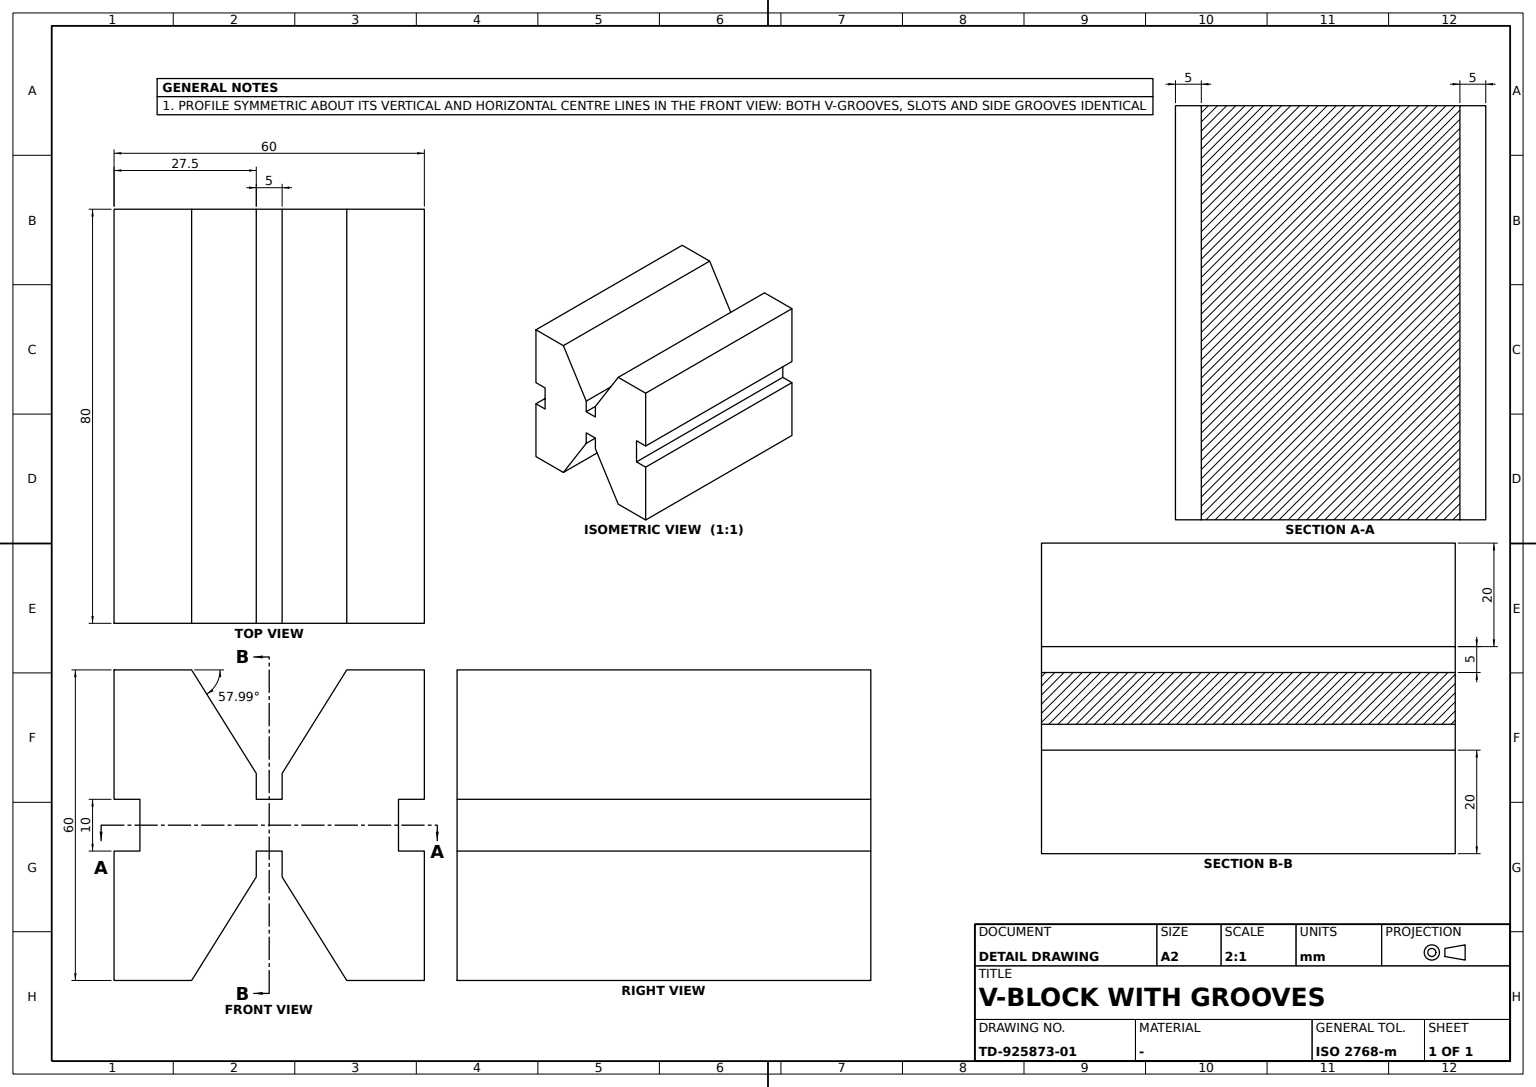
ISO-10303-21;
HEADER;
FILE_DESCRIPTION((''),'2;1');
FILE_NAME('','',(''),(''),'','','');
FILE_SCHEMA(('AUTOMOTIVE_DESIGN'));
ENDSEC;
DATA;
#1=APPLICATION_CONTEXT('');
#2=PRODUCT_CONTEXT('',#1,'mechanical');
#3=PRODUCT('','','',(#2));
#4=PRODUCT_DEFINITION_FORMATION('','',#3);
#5=PRODUCT_DEFINITION_CONTEXT('',#1,'design');
#6=PRODUCT_DEFINITION('','',#4,#5);
#7=PRODUCT_DEFINITION_SHAPE('','',#6);
#8=(LENGTH_UNIT()NAMED_UNIT(*)SI_UNIT(.MILLI.,.METRE.));
#9=(NAMED_UNIT(*)PLANE_ANGLE_UNIT()SI_UNIT($,.RADIAN.));
#10=(NAMED_UNIT(*)SI_UNIT($,.STERADIAN.)SOLID_ANGLE_UNIT());
#11=UNCERTAINTY_MEASURE_WITH_UNIT(LENGTH_MEASURE(1.E-05),#8,'distance_accuracy_value','');
#12=(GEOMETRIC_REPRESENTATION_CONTEXT(3)GLOBAL_UNCERTAINTY_ASSIGNED_CONTEXT((#11))GLOBAL_UNIT_ASSIGNED_CONTEXT((#8,#9,#10))REPRESENTATION_CONTEXT('',''));
#13=CARTESIAN_POINT('',(-40.,-2.5,10.));
#14=VERTEX_POINT('',#13);
#15=CARTESIAN_POINT('',(40.,-2.5,10.));
#16=VERTEX_POINT('',#15);
#17=CARTESIAN_POINT('',(0.,-2.5,10.));
#18=DIRECTION('',(1.,0.,0.));
#19=VECTOR('',#18,1000.);
#20=LINE('',#17,#19);
#21=EDGE_CURVE('',#14,#16,#20,.T.);
#22=ORIENTED_EDGE('',*,*,#21,.F.);
#23=CARTESIAN_POINT('',(-40.,-15.,30.));
#24=VERTEX_POINT('',#23);
#25=CARTESIAN_POINT('',(-40.,-8.75,20.));
#26=DIRECTION('',(0.,0.52999894,-0.847998304));
#27=VECTOR('',#26,1000.);
#28=LINE('',#25,#27);
#29=EDGE_CURVE('',#24,#14,#28,.T.);
#30=ORIENTED_EDGE('',*,*,#29,.F.);
#31=CARTESIAN_POINT('',(40.,-15.,30.));
#32=VERTEX_POINT('',#31);
#33=CARTESIAN_POINT('',(0.,-15.,30.));
#34=LINE('',#33,#19);
#35=EDGE_CURVE('',#24,#32,#34,.T.);
#36=ORIENTED_EDGE('',*,*,#35,.T.);
#37=CARTESIAN_POINT('',(40.,-8.75,20.));
#38=LINE('',#37,#27);
#39=EDGE_CURVE('',#32,#16,#38,.T.);
#40=ORIENTED_EDGE('',*,*,#39,.T.);
#41=EDGE_LOOP('',(#22,#30,#36,#40));
#42=FACE_OUTER_BOUND('',#41,.T.);
#43=DIRECTION('',(0.,0.847998304,0.52999894));
#44=DIRECTION('',(0.,-0.52999894,0.847998304));
#45=AXIS2_PLACEMENT_3D('',#17,#43,#44);
#46=PLANE('',#45);
#47=ADVANCED_FACE('',(#42),#46,.T.);
#48=CARTESIAN_POINT('',(-40.,-15.,-30.));
#49=VERTEX_POINT('',#48);
#50=CARTESIAN_POINT('',(40.,-15.,-30.));
#51=VERTEX_POINT('',#50);
#52=CARTESIAN_POINT('',(0.,-15.,-30.));
#53=LINE('',#52,#19);
#54=EDGE_CURVE('',#49,#51,#53,.T.);
#55=ORIENTED_EDGE('',*,*,#54,.T.);
#56=CARTESIAN_POINT('',(40.,-30.,-30.));
#57=VERTEX_POINT('',#56);
#58=CARTESIAN_POINT('',(40.,-22.5,-30.));
#59=DIRECTION('',(0.,-1.,0.));
#60=VECTOR('',#59,1000.);
#61=LINE('',#58,#60);
#62=EDGE_CURVE('',#51,#57,#61,.T.);
#63=ORIENTED_EDGE('',*,*,#62,.T.);
#64=CARTESIAN_POINT('',(-40.,-30.,-30.));
#65=VERTEX_POINT('',#64);
#66=CARTESIAN_POINT('',(0.,-30.,-30.));
#67=LINE('',#66,#19);
#68=EDGE_CURVE('',#65,#57,#67,.T.);
#69=ORIENTED_EDGE('',*,*,#68,.F.);
#70=CARTESIAN_POINT('',(-40.,-22.5,-30.));
#71=LINE('',#70,#60);
#72=EDGE_CURVE('',#49,#65,#71,.T.);
#73=ORIENTED_EDGE('',*,*,#72,.F.);
#74=EDGE_LOOP('',(#55,#63,#69,#73));
#75=FACE_OUTER_BOUND('',#74,.T.);
#76=CARTESIAN_POINT('',(0.,30.,-30.));
#77=DIRECTION('',(0.,0.,1.));
#78=AXIS2_PLACEMENT_3D('',#76,#77,#59);
#79=PLANE('',#78);
#80=ADVANCED_FACE('',(#75),#79,.F.);
#81=CARTESIAN_POINT('',(-40.,2.5,10.));
#82=VERTEX_POINT('',#81);
#83=CARTESIAN_POINT('',(-40.,2.5,5.));
#84=VERTEX_POINT('',#83);
#85=CARTESIAN_POINT('',(-40.,2.5,7.5));
#86=DIRECTION('',(0.,0.,-1.));
#87=VECTOR('',#86,1000.);
#88=LINE('',#85,#87);
#89=EDGE_CURVE('',#82,#84,#88,.T.);
#90=ORIENTED_EDGE('',*,*,#89,.T.);
#91=CARTESIAN_POINT('',(40.,2.5,5.));
#92=VERTEX_POINT('',#91);
#93=CARTESIAN_POINT('',(0.,2.5,5.));
#94=LINE('',#93,#19);
#95=EDGE_CURVE('',#84,#92,#94,.T.);
#96=ORIENTED_EDGE('',*,*,#95,.T.);
#97=CARTESIAN_POINT('',(40.,2.5,10.));
#98=VERTEX_POINT('',#97);
#99=CARTESIAN_POINT('',(40.,2.5,7.5));
#100=LINE('',#99,#87);
#101=EDGE_CURVE('',#98,#92,#100,.T.);
#102=ORIENTED_EDGE('',*,*,#101,.F.);
#103=CARTESIAN_POINT('',(0.,2.5,10.));
#104=LINE('',#103,#19);
#105=EDGE_CURVE('',#82,#98,#104,.T.);
#106=ORIENTED_EDGE('',*,*,#105,.F.);
#107=EDGE_LOOP('',(#90,#96,#102,#106));
#108=FACE_OUTER_BOUND('',#107,.T.);
#109=DIRECTION('',(0.,1.,0.));
#110=AXIS2_PLACEMENT_3D('',#93,#109,#77);
#111=PLANE('',#110);
#112=ADVANCED_FACE('',(#108),#111,.F.);
#113=CARTESIAN_POINT('',(-40.,-2.5,5.));
#114=VERTEX_POINT('',#113);
#115=CARTESIAN_POINT('',(-40.,0.,5.));
#116=VECTOR('',#109,1000.);
#117=LINE('',#115,#116);
#118=EDGE_CURVE('',#114,#84,#117,.T.);
#119=ORIENTED_EDGE('',*,*,#118,.F.);
#120=CARTESIAN_POINT('',(40.,-2.5,5.));
#121=VERTEX_POINT('',#120);
#122=CARTESIAN_POINT('',(0.,-2.5,5.));
#123=LINE('',#122,#19);
#124=EDGE_CURVE('',#114,#121,#123,.T.);
#125=ORIENTED_EDGE('',*,*,#124,.T.);
#126=CARTESIAN_POINT('',(40.,0.,5.));
#127=LINE('',#126,#116);
#128=EDGE_CURVE('',#121,#92,#127,.T.);
#129=ORIENTED_EDGE('',*,*,#128,.T.);
#130=ORIENTED_EDGE('',*,*,#95,.F.);
#131=EDGE_LOOP('',(#119,#125,#129,#130));
#132=FACE_OUTER_BOUND('',#131,.T.);
#133=CARTESIAN_POINT('',(0.,0.,5.));
#134=AXIS2_PLACEMENT_3D('',#133,#86,#109);
#135=PLANE('',#134);
#136=ADVANCED_FACE('',(#132),#135,.F.);
#137=CARTESIAN_POINT('',(-40.,-30.,-5.));
#138=VERTEX_POINT('',#137);
#139=CARTESIAN_POINT('',(-40.,-25.,-5.));
#140=VERTEX_POINT('',#139);
#141=CARTESIAN_POINT('',(-40.,-27.5,-5.));
#142=LINE('',#141,#116);
#143=EDGE_CURVE('',#138,#140,#142,.T.);
#144=ORIENTED_EDGE('',*,*,#143,.F.);
#145=CARTESIAN_POINT('',(40.,-30.,-5.));
#146=VERTEX_POINT('',#145);
#147=CARTESIAN_POINT('',(0.,-30.,-5.));
#148=LINE('',#147,#19);
#149=EDGE_CURVE('',#138,#146,#148,.T.);
#150=ORIENTED_EDGE('',*,*,#149,.T.);
#151=CARTESIAN_POINT('',(40.,-25.,-5.));
#152=VERTEX_POINT('',#151);
#153=CARTESIAN_POINT('',(40.,-27.5,-5.));
#154=LINE('',#153,#116);
#155=EDGE_CURVE('',#146,#152,#154,.T.);
#156=ORIENTED_EDGE('',*,*,#155,.T.);
#157=CARTESIAN_POINT('',(0.,-25.,-5.));
#158=LINE('',#157,#19);
#159=EDGE_CURVE('',#140,#152,#158,.T.);
#160=ORIENTED_EDGE('',*,*,#159,.F.);
#161=EDGE_LOOP('',(#144,#150,#156,#160));
#162=FACE_OUTER_BOUND('',#161,.T.);
#163=CARTESIAN_POINT('',(0.,0.,-5.));
#164=AXIS2_PLACEMENT_3D('',#163,#86,#109);
#165=PLANE('',#164);
#166=ADVANCED_FACE('',(#162),#165,.F.);
#167=CARTESIAN_POINT('',(-40.,15.,-30.));
#168=VERTEX_POINT('',#167);
#169=CARTESIAN_POINT('',(-40.,30.,-30.));
#170=VERTEX_POINT('',#169);
#171=CARTESIAN_POINT('',(-40.,22.5,-30.));
#172=LINE('',#171,#116);
#173=EDGE_CURVE('',#168,#170,#172,.T.);
#174=ORIENTED_EDGE('',*,*,#173,.T.);
#175=CARTESIAN_POINT('',(40.,30.,-30.));
#176=VERTEX_POINT('',#175);
#177=LINE('',#76,#19);
#178=EDGE_CURVE('',#170,#176,#177,.T.);
#179=ORIENTED_EDGE('',*,*,#178,.T.);
#180=CARTESIAN_POINT('',(40.,15.,-30.));
#181=VERTEX_POINT('',#180);
#182=CARTESIAN_POINT('',(40.,22.5,-30.));
#183=LINE('',#182,#116);
#184=EDGE_CURVE('',#181,#176,#183,.T.);
#185=ORIENTED_EDGE('',*,*,#184,.F.);
#186=CARTESIAN_POINT('',(0.,15.,-30.));
#187=LINE('',#186,#19);
#188=EDGE_CURVE('',#168,#181,#187,.T.);
#189=ORIENTED_EDGE('',*,*,#188,.F.);
#190=EDGE_LOOP('',(#174,#179,#185,#189));
#191=FACE_OUTER_BOUND('',#190,.T.);
#192=ADVANCED_FACE('',(#191),#79,.F.);
#193=ORIENTED_EDGE('',*,*,#124,.F.);
#194=CARTESIAN_POINT('',(-40.,-2.5,7.5));
#195=LINE('',#194,#87);
#196=EDGE_CURVE('',#14,#114,#195,.T.);
#197=ORIENTED_EDGE('',*,*,#196,.F.);
#198=ORIENTED_EDGE('',*,*,#21,.T.);
#199=CARTESIAN_POINT('',(40.,-2.5,7.5));
#200=LINE('',#199,#87);
#201=EDGE_CURVE('',#16,#121,#200,.T.);
#202=ORIENTED_EDGE('',*,*,#201,.T.);
#203=EDGE_LOOP('',(#193,#197,#198,#202));
#204=FACE_OUTER_BOUND('',#203,.T.);
#205=AXIS2_PLACEMENT_3D('',#122,#109,#77);
#206=PLANE('',#205);
#207=ADVANCED_FACE('',(#204),#206,.T.);
#208=CARTESIAN_POINT('',(-40.,30.,5.));
#209=VERTEX_POINT('',#208);
#210=CARTESIAN_POINT('',(-40.,30.,30.));
#211=VERTEX_POINT('',#210);
#212=CARTESIAN_POINT('',(-40.,30.,17.5));
#213=VECTOR('',#77,1000.);
#214=LINE('',#212,#213);
#215=EDGE_CURVE('',#209,#211,#214,.T.);
#216=ORIENTED_EDGE('',*,*,#215,.T.);
#217=CARTESIAN_POINT('',(40.,30.,30.));
#218=VERTEX_POINT('',#217);
#219=CARTESIAN_POINT('',(0.,30.,30.));
#220=LINE('',#219,#19);
#221=EDGE_CURVE('',#211,#218,#220,.T.);
#222=ORIENTED_EDGE('',*,*,#221,.T.);
#223=CARTESIAN_POINT('',(40.,30.,5.));
#224=VERTEX_POINT('',#223);
#225=CARTESIAN_POINT('',(40.,30.,17.5));
#226=LINE('',#225,#213);
#227=EDGE_CURVE('',#224,#218,#226,.T.);
#228=ORIENTED_EDGE('',*,*,#227,.F.);
#229=CARTESIAN_POINT('',(0.,30.,5.));
#230=LINE('',#229,#19);
#231=EDGE_CURVE('',#209,#224,#230,.T.);
#232=ORIENTED_EDGE('',*,*,#231,.F.);
#233=EDGE_LOOP('',(#216,#222,#228,#232));
#234=FACE_OUTER_BOUND('',#233,.T.);
#235=CARTESIAN_POINT('',(0.,30.,-5.));
#236=AXIS2_PLACEMENT_3D('',#235,#59,#86);
#237=PLANE('',#236);
#238=ADVANCED_FACE('',(#234),#237,.F.);
#239=CARTESIAN_POINT('',(-40.,15.,30.));
#240=VERTEX_POINT('',#239);
#241=CARTESIAN_POINT('',(40.,15.,30.));
#242=VERTEX_POINT('',#241);
#243=CARTESIAN_POINT('',(0.,15.,30.));
#244=LINE('',#243,#19);
#245=EDGE_CURVE('',#240,#242,#244,.T.);
#246=ORIENTED_EDGE('',*,*,#245,.T.);
#247=CARTESIAN_POINT('',(40.,22.5,30.));
#248=LINE('',#247,#60);
#249=EDGE_CURVE('',#218,#242,#248,.T.);
#250=ORIENTED_EDGE('',*,*,#249,.F.);
#251=ORIENTED_EDGE('',*,*,#221,.F.);
#252=CARTESIAN_POINT('',(-40.,22.5,30.));
#253=LINE('',#252,#60);
#254=EDGE_CURVE('',#211,#240,#253,.T.);
#255=ORIENTED_EDGE('',*,*,#254,.T.);
#256=EDGE_LOOP('',(#246,#250,#251,#255));
#257=FACE_OUTER_BOUND('',#256,.T.);
#258=AXIS2_PLACEMENT_3D('',#243,#86,#109);
#259=PLANE('',#258);
#260=ADVANCED_FACE('',(#257),#259,.F.);
#261=CARTESIAN_POINT('',(40.,25.,5.));
#262=VERTEX_POINT('',#261);
#263=CARTESIAN_POINT('',(40.,27.5,5.));
#264=LINE('',#263,#116);
#265=EDGE_CURVE('',#262,#224,#264,.T.);
#266=ORIENTED_EDGE('',*,*,#265,.F.);
#267=CARTESIAN_POINT('',(-40.,25.,5.));
#268=VERTEX_POINT('',#267);
#269=CARTESIAN_POINT('',(0.,25.,5.));
#270=LINE('',#269,#19);
#271=EDGE_CURVE('',#268,#262,#270,.T.);
#272=ORIENTED_EDGE('',*,*,#271,.F.);
#273=CARTESIAN_POINT('',(-40.,27.5,5.));
#274=LINE('',#273,#116);
#275=EDGE_CURVE('',#268,#209,#274,.T.);
#276=ORIENTED_EDGE('',*,*,#275,.T.);
#277=ORIENTED_EDGE('',*,*,#231,.T.);
#278=EDGE_LOOP('',(#266,#272,#276,#277));
#279=FACE_OUTER_BOUND('',#278,.T.);
#280=ADVANCED_FACE('',(#279),#135,.T.);
#281=ORIENTED_EDGE('',*,*,#178,.F.);
#282=CARTESIAN_POINT('',(-40.,30.,-5.));
#283=VERTEX_POINT('',#282);
#284=CARTESIAN_POINT('',(-40.,30.,-17.5));
#285=LINE('',#284,#213);
#286=EDGE_CURVE('',#170,#283,#285,.T.);
#287=ORIENTED_EDGE('',*,*,#286,.T.);
#288=CARTESIAN_POINT('',(40.,30.,-5.));
#289=VERTEX_POINT('',#288);
#290=LINE('',#235,#19);
#291=EDGE_CURVE('',#283,#289,#290,.T.);
#292=ORIENTED_EDGE('',*,*,#291,.T.);
#293=CARTESIAN_POINT('',(40.,30.,-17.5));
#294=LINE('',#293,#213);
#295=EDGE_CURVE('',#176,#289,#294,.T.);
#296=ORIENTED_EDGE('',*,*,#295,.F.);
#297=EDGE_LOOP('',(#281,#287,#292,#296));
#298=FACE_OUTER_BOUND('',#297,.T.);
#299=ADVANCED_FACE('',(#298),#237,.F.);
#300=CARTESIAN_POINT('',(-40.,25.,-5.));
#301=VERTEX_POINT('',#300);
#302=CARTESIAN_POINT('',(40.,25.,-5.));
#303=VERTEX_POINT('',#302);
#304=CARTESIAN_POINT('',(0.,25.,-5.));
#305=LINE('',#304,#19);
#306=EDGE_CURVE('',#301,#303,#305,.T.);
#307=ORIENTED_EDGE('',*,*,#306,.F.);
#308=CARTESIAN_POINT('',(-40.,25.,0.));
#309=LINE('',#308,#213);
#310=EDGE_CURVE('',#301,#268,#309,.T.);
#311=ORIENTED_EDGE('',*,*,#310,.T.);
#312=ORIENTED_EDGE('',*,*,#271,.T.);
#313=CARTESIAN_POINT('',(40.,25.,0.));
#314=LINE('',#313,#213);
#315=EDGE_CURVE('',#303,#262,#314,.T.);
#316=ORIENTED_EDGE('',*,*,#315,.F.);
#317=EDGE_LOOP('',(#307,#311,#312,#316));
#318=FACE_OUTER_BOUND('',#317,.T.);
#319=AXIS2_PLACEMENT_3D('',#269,#59,#86);
#320=PLANE('',#319);
#321=ADVANCED_FACE('',(#318),#320,.F.);
#322=CARTESIAN_POINT('',(-40.,-30.,30.));
#323=VERTEX_POINT('',#322);
#324=CARTESIAN_POINT('',(40.,-30.,30.));
#325=VERTEX_POINT('',#324);
#326=CARTESIAN_POINT('',(0.,-30.,30.));
#327=LINE('',#326,#19);
#328=EDGE_CURVE('',#323,#325,#327,.T.);
#329=ORIENTED_EDGE('',*,*,#328,.F.);
#330=CARTESIAN_POINT('',(-40.,-30.,5.));
#331=VERTEX_POINT('',#330);
#332=CARTESIAN_POINT('',(-40.,-30.,17.5));
#333=LINE('',#332,#213);
#334=EDGE_CURVE('',#331,#323,#333,.T.);
#335=ORIENTED_EDGE('',*,*,#334,.F.);
#336=CARTESIAN_POINT('',(40.,-30.,5.));
#337=VERTEX_POINT('',#336);
#338=CARTESIAN_POINT('',(0.,-30.,5.));
#339=LINE('',#338,#19);
#340=EDGE_CURVE('',#331,#337,#339,.T.);
#341=ORIENTED_EDGE('',*,*,#340,.T.);
#342=CARTESIAN_POINT('',(40.,-30.,17.5));
#343=LINE('',#342,#213);
#344=EDGE_CURVE('',#337,#325,#343,.T.);
#345=ORIENTED_EDGE('',*,*,#344,.T.);
#346=EDGE_LOOP('',(#329,#335,#341,#345));
#347=FACE_OUTER_BOUND('',#346,.T.);
#348=AXIS2_PLACEMENT_3D('',#147,#59,#86);
#349=PLANE('',#348);
#350=ADVANCED_FACE('',(#347),#349,.T.);
#351=ORIENTED_EDGE('',*,*,#128,.F.);
#352=ORIENTED_EDGE('',*,*,#201,.F.);
#353=ORIENTED_EDGE('',*,*,#39,.F.);
#354=CARTESIAN_POINT('',(40.,-22.5,30.));
#355=LINE('',#354,#116);
#356=EDGE_CURVE('',#325,#32,#355,.T.);
#357=ORIENTED_EDGE('',*,*,#356,.F.);
#358=ORIENTED_EDGE('',*,*,#344,.F.);
#359=CARTESIAN_POINT('',(40.,-25.,5.));
#360=VERTEX_POINT('',#359);
#361=CARTESIAN_POINT('',(40.,-27.5,5.));
#362=LINE('',#361,#60);
#363=EDGE_CURVE('',#360,#337,#362,.T.);
#364=ORIENTED_EDGE('',*,*,#363,.F.);
#365=CARTESIAN_POINT('',(40.,-25.,0.));
#366=LINE('',#365,#213);
#367=EDGE_CURVE('',#152,#360,#366,.T.);
#368=ORIENTED_EDGE('',*,*,#367,.F.);
#369=ORIENTED_EDGE('',*,*,#155,.F.);
#370=CARTESIAN_POINT('',(40.,-30.,-17.5));
#371=LINE('',#370,#213);
#372=EDGE_CURVE('',#57,#146,#371,.T.);
#373=ORIENTED_EDGE('',*,*,#372,.F.);
#374=ORIENTED_EDGE('',*,*,#62,.F.);
#375=CARTESIAN_POINT('',(40.,-2.5,-10.));
#376=VERTEX_POINT('',#375);
#377=CARTESIAN_POINT('',(40.,-8.75,-20.));
#378=DIRECTION('',(0.,-0.52999894,-0.847998304));
#379=VECTOR('',#378,1000.);
#380=LINE('',#377,#379);
#381=EDGE_CURVE('',#376,#51,#380,.T.);
#382=ORIENTED_EDGE('',*,*,#381,.F.);
#383=CARTESIAN_POINT('',(40.,-2.5,-5.));
#384=VERTEX_POINT('',#383);
#385=CARTESIAN_POINT('',(40.,-2.5,-7.5));
#386=LINE('',#385,#87);
#387=EDGE_CURVE('',#384,#376,#386,.T.);
#388=ORIENTED_EDGE('',*,*,#387,.F.);
#389=CARTESIAN_POINT('',(40.,2.5,-5.));
#390=VERTEX_POINT('',#389);
#391=CARTESIAN_POINT('',(40.,0.,-5.));
#392=LINE('',#391,#60);
#393=EDGE_CURVE('',#390,#384,#392,.T.);
#394=ORIENTED_EDGE('',*,*,#393,.F.);
#395=CARTESIAN_POINT('',(40.,2.5,-10.));
#396=VERTEX_POINT('',#395);
#397=CARTESIAN_POINT('',(40.,2.5,-7.5));
#398=LINE('',#397,#87);
#399=EDGE_CURVE('',#390,#396,#398,.T.);
#400=ORIENTED_EDGE('',*,*,#399,.T.);
#401=CARTESIAN_POINT('',(40.,8.75,-20.));
#402=LINE('',#401,#27);
#403=EDGE_CURVE('',#396,#181,#402,.T.);
#404=ORIENTED_EDGE('',*,*,#403,.T.);
#405=ORIENTED_EDGE('',*,*,#184,.T.);
#406=ORIENTED_EDGE('',*,*,#295,.T.);
#407=CARTESIAN_POINT('',(40.,27.5,-5.));
#408=LINE('',#407,#60);
#409=EDGE_CURVE('',#289,#303,#408,.T.);
#410=ORIENTED_EDGE('',*,*,#409,.T.);
#411=ORIENTED_EDGE('',*,*,#315,.T.);
#412=ORIENTED_EDGE('',*,*,#265,.T.);
#413=ORIENTED_EDGE('',*,*,#227,.T.);
#414=ORIENTED_EDGE('',*,*,#249,.T.);
#415=CARTESIAN_POINT('',(40.,8.75,20.));
#416=LINE('',#415,#379);
#417=EDGE_CURVE('',#242,#98,#416,.T.);
#418=ORIENTED_EDGE('',*,*,#417,.T.);
#419=ORIENTED_EDGE('',*,*,#101,.T.);
#420=EDGE_LOOP('',(#351,#352,#353,#357,#358,#364,#368,#369,#373,#374,#382,#388,#394,#400,#404,#405,#406,#410,#411,#412,#413,#414,#418,#419));
#421=FACE_OUTER_BOUND('',#420,.T.);
#422=CARTESIAN_POINT('',(40.,0.,0.));
#423=AXIS2_PLACEMENT_3D('',#422,#18,#109);
#424=PLANE('',#423);
#425=ADVANCED_FACE('',(#421),#424,.T.);
#426=CARTESIAN_POINT('',(-40.,2.5,-5.));
#427=VERTEX_POINT('',#426);
#428=CARTESIAN_POINT('',(-40.,-2.5,-5.));
#429=VERTEX_POINT('',#428);
#430=CARTESIAN_POINT('',(-40.,0.,-5.));
#431=LINE('',#430,#60);
#432=EDGE_CURVE('',#427,#429,#431,.T.);
#433=ORIENTED_EDGE('',*,*,#432,.T.);
#434=CARTESIAN_POINT('',(-40.,-2.5,-10.));
#435=VERTEX_POINT('',#434);
#436=CARTESIAN_POINT('',(-40.,-2.5,-7.5));
#437=LINE('',#436,#87);
#438=EDGE_CURVE('',#429,#435,#437,.T.);
#439=ORIENTED_EDGE('',*,*,#438,.T.);
#440=CARTESIAN_POINT('',(-40.,-8.75,-20.));
#441=LINE('',#440,#379);
#442=EDGE_CURVE('',#435,#49,#441,.T.);
#443=ORIENTED_EDGE('',*,*,#442,.T.);
#444=ORIENTED_EDGE('',*,*,#72,.T.);
#445=CARTESIAN_POINT('',(-40.,-30.,-17.5));
#446=LINE('',#445,#213);
#447=EDGE_CURVE('',#65,#138,#446,.T.);
#448=ORIENTED_EDGE('',*,*,#447,.T.);
#449=ORIENTED_EDGE('',*,*,#143,.T.);
#450=CARTESIAN_POINT('',(-40.,-25.,5.));
#451=VERTEX_POINT('',#450);
#452=CARTESIAN_POINT('',(-40.,-25.,0.));
#453=LINE('',#452,#213);
#454=EDGE_CURVE('',#140,#451,#453,.T.);
#455=ORIENTED_EDGE('',*,*,#454,.T.);
#456=CARTESIAN_POINT('',(-40.,-27.5,5.));
#457=LINE('',#456,#60);
#458=EDGE_CURVE('',#451,#331,#457,.T.);
#459=ORIENTED_EDGE('',*,*,#458,.T.);
#460=ORIENTED_EDGE('',*,*,#334,.T.);
#461=CARTESIAN_POINT('',(-40.,-22.5,30.));
#462=LINE('',#461,#116);
#463=EDGE_CURVE('',#323,#24,#462,.T.);
#464=ORIENTED_EDGE('',*,*,#463,.T.);
#465=ORIENTED_EDGE('',*,*,#29,.T.);
#466=ORIENTED_EDGE('',*,*,#196,.T.);
#467=ORIENTED_EDGE('',*,*,#118,.T.);
#468=ORIENTED_EDGE('',*,*,#89,.F.);
#469=CARTESIAN_POINT('',(-40.,8.75,20.));
#470=LINE('',#469,#379);
#471=EDGE_CURVE('',#240,#82,#470,.T.);
#472=ORIENTED_EDGE('',*,*,#471,.F.);
#473=ORIENTED_EDGE('',*,*,#254,.F.);
#474=ORIENTED_EDGE('',*,*,#215,.F.);
#475=ORIENTED_EDGE('',*,*,#275,.F.);
#476=ORIENTED_EDGE('',*,*,#310,.F.);
#477=CARTESIAN_POINT('',(-40.,27.5,-5.));
#478=LINE('',#477,#60);
#479=EDGE_CURVE('',#283,#301,#478,.T.);
#480=ORIENTED_EDGE('',*,*,#479,.F.);
#481=ORIENTED_EDGE('',*,*,#286,.F.);
#482=ORIENTED_EDGE('',*,*,#173,.F.);
#483=CARTESIAN_POINT('',(-40.,2.5,-10.));
#484=VERTEX_POINT('',#483);
#485=CARTESIAN_POINT('',(-40.,8.75,-20.));
#486=LINE('',#485,#27);
#487=EDGE_CURVE('',#484,#168,#486,.T.);
#488=ORIENTED_EDGE('',*,*,#487,.F.);
#489=CARTESIAN_POINT('',(-40.,2.5,-7.5));
#490=LINE('',#489,#87);
#491=EDGE_CURVE('',#427,#484,#490,.T.);
#492=ORIENTED_EDGE('',*,*,#491,.F.);
#493=EDGE_LOOP('',(#433,#439,#443,#444,#448,#449,#455,#459,#460,#464,#465,#466,#467,#468,#472,#473,#474,#475,#476,#480,#481,#482,#488,#492));
#494=FACE_OUTER_BOUND('',#493,.T.);
#495=CARTESIAN_POINT('',(-40.,0.,0.));
#496=AXIS2_PLACEMENT_3D('',#495,#18,#109);
#497=PLANE('',#496);
#498=ADVANCED_FACE('',(#494),#497,.F.);
#499=ORIENTED_EDGE('',*,*,#417,.F.);
#500=ORIENTED_EDGE('',*,*,#245,.F.);
#501=ORIENTED_EDGE('',*,*,#471,.T.);
#502=ORIENTED_EDGE('',*,*,#105,.T.);
#503=EDGE_LOOP('',(#499,#500,#501,#502));
#504=FACE_OUTER_BOUND('',#503,.T.);
#505=DIRECTION('',(0.,0.847998304,-0.52999894));
#506=DIRECTION('',(0.,0.52999894,0.847998304));
#507=AXIS2_PLACEMENT_3D('',#103,#505,#506);
#508=PLANE('',#507);
#509=ADVANCED_FACE('',(#504),#508,.F.);
#510=ORIENTED_EDGE('',*,*,#372,.T.);
#511=ORIENTED_EDGE('',*,*,#149,.F.);
#512=ORIENTED_EDGE('',*,*,#447,.F.);
#513=ORIENTED_EDGE('',*,*,#68,.T.);
#514=EDGE_LOOP('',(#510,#511,#512,#513));
#515=FACE_OUTER_BOUND('',#514,.T.);
#516=ADVANCED_FACE('',(#515),#349,.T.);
#517=ORIENTED_EDGE('',*,*,#381,.T.);
#518=ORIENTED_EDGE('',*,*,#54,.F.);
#519=ORIENTED_EDGE('',*,*,#442,.F.);
#520=CARTESIAN_POINT('',(0.,-2.5,-10.));
#521=LINE('',#520,#19);
#522=EDGE_CURVE('',#435,#376,#521,.T.);
#523=ORIENTED_EDGE('',*,*,#522,.T.);
#524=EDGE_LOOP('',(#517,#518,#519,#523));
#525=FACE_OUTER_BOUND('',#524,.T.);
#526=DIRECTION('',(0.,-0.847998304,0.52999894));
#527=AXIS2_PLACEMENT_3D('',#520,#526,#378);
#528=PLANE('',#527);
#529=ADVANCED_FACE('',(#525),#528,.F.);
#530=CARTESIAN_POINT('',(0.,2.5,-5.));
#531=LINE('',#530,#19);
#532=EDGE_CURVE('',#427,#390,#531,.T.);
#533=ORIENTED_EDGE('',*,*,#532,.T.);
#534=ORIENTED_EDGE('',*,*,#393,.T.);
#535=CARTESIAN_POINT('',(0.,-2.5,-5.));
#536=LINE('',#535,#19);
#537=EDGE_CURVE('',#429,#384,#536,.T.);
#538=ORIENTED_EDGE('',*,*,#537,.F.);
#539=ORIENTED_EDGE('',*,*,#432,.F.);
#540=EDGE_LOOP('',(#533,#534,#538,#539));
#541=FACE_OUTER_BOUND('',#540,.T.);
#542=ADVANCED_FACE('',(#541),#165,.T.);
#543=ORIENTED_EDGE('',*,*,#399,.F.);
#544=ORIENTED_EDGE('',*,*,#532,.F.);
#545=ORIENTED_EDGE('',*,*,#491,.T.);
#546=CARTESIAN_POINT('',(0.,2.5,-10.));
#547=LINE('',#546,#19);
#548=EDGE_CURVE('',#484,#396,#547,.T.);
#549=ORIENTED_EDGE('',*,*,#548,.T.);
#550=EDGE_LOOP('',(#543,#544,#545,#549));
#551=FACE_OUTER_BOUND('',#550,.T.);
#552=ADVANCED_FACE('',(#551),#111,.F.);
#553=ORIENTED_EDGE('',*,*,#367,.T.);
#554=CARTESIAN_POINT('',(0.,-25.,5.));
#555=LINE('',#554,#19);
#556=EDGE_CURVE('',#451,#360,#555,.T.);
#557=ORIENTED_EDGE('',*,*,#556,.F.);
#558=ORIENTED_EDGE('',*,*,#454,.F.);
#559=ORIENTED_EDGE('',*,*,#159,.T.);
#560=EDGE_LOOP('',(#553,#557,#558,#559));
#561=FACE_OUTER_BOUND('',#560,.T.);
#562=AXIS2_PLACEMENT_3D('',#554,#59,#86);
#563=PLANE('',#562);
#564=ADVANCED_FACE('',(#561),#563,.T.);
#565=ORIENTED_EDGE('',*,*,#356,.T.);
#566=ORIENTED_EDGE('',*,*,#35,.F.);
#567=ORIENTED_EDGE('',*,*,#463,.F.);
#568=ORIENTED_EDGE('',*,*,#328,.T.);
#569=EDGE_LOOP('',(#565,#566,#567,#568));
#570=FACE_OUTER_BOUND('',#569,.T.);
#571=ADVANCED_FACE('',(#570),#259,.F.);
#572=ORIENTED_EDGE('',*,*,#458,.F.);
#573=ORIENTED_EDGE('',*,*,#556,.T.);
#574=ORIENTED_EDGE('',*,*,#363,.T.);
#575=ORIENTED_EDGE('',*,*,#340,.F.);
#576=EDGE_LOOP('',(#572,#573,#574,#575));
#577=FACE_OUTER_BOUND('',#576,.T.);
#578=ADVANCED_FACE('',(#577),#135,.T.);
#579=ORIENTED_EDGE('',*,*,#438,.F.);
#580=ORIENTED_EDGE('',*,*,#537,.T.);
#581=ORIENTED_EDGE('',*,*,#387,.T.);
#582=ORIENTED_EDGE('',*,*,#522,.F.);
#583=EDGE_LOOP('',(#579,#580,#581,#582));
#584=FACE_OUTER_BOUND('',#583,.T.);
#585=ADVANCED_FACE('',(#584),#206,.T.);
#586=ORIENTED_EDGE('',*,*,#188,.T.);
#587=ORIENTED_EDGE('',*,*,#403,.F.);
#588=ORIENTED_EDGE('',*,*,#548,.F.);
#589=ORIENTED_EDGE('',*,*,#487,.T.);
#590=EDGE_LOOP('',(#586,#587,#588,#589));
#591=FACE_OUTER_BOUND('',#590,.T.);
#592=DIRECTION('',(0.,-0.847998304,-0.52999894));
#593=AXIS2_PLACEMENT_3D('',#546,#592,#26);
#594=PLANE('',#593);
#595=ADVANCED_FACE('',(#591),#594,.T.);
#596=ORIENTED_EDGE('',*,*,#479,.T.);
#597=ORIENTED_EDGE('',*,*,#306,.T.);
#598=ORIENTED_EDGE('',*,*,#409,.F.);
#599=ORIENTED_EDGE('',*,*,#291,.F.);
#600=EDGE_LOOP('',(#596,#597,#598,#599));
#601=FACE_OUTER_BOUND('',#600,.T.);
#602=ADVANCED_FACE('',(#601),#165,.F.);
#603=CLOSED_SHELL('',(#47,#80,#112,#136,#166,#192,#207,#238,#260,#280,#299,#321,#350,#425,#498,#509,#516,#529,#542,#552,#564,#571,#578,#585,#595,#602));
#604=MANIFOLD_SOLID_BREP('',#603);
#605=ADVANCED_BREP_SHAPE_REPRESENTATION('',(#604),#12);
#606=SHAPE_DEFINITION_REPRESENTATION(#7,#605);
ENDSEC;
END-ISO-10303-21;
